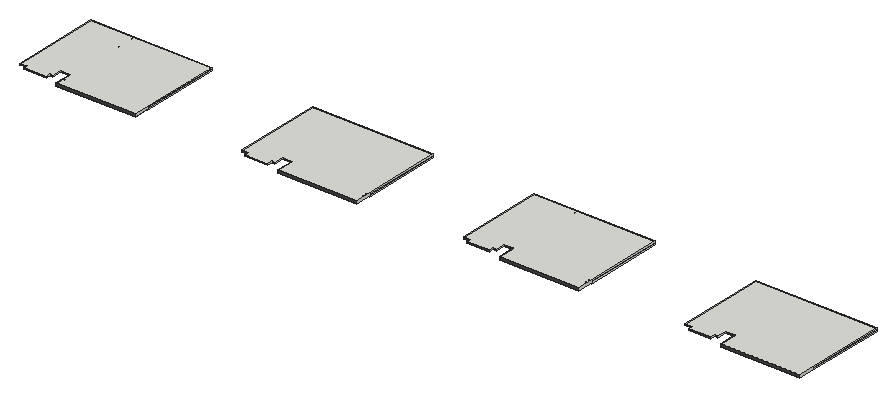
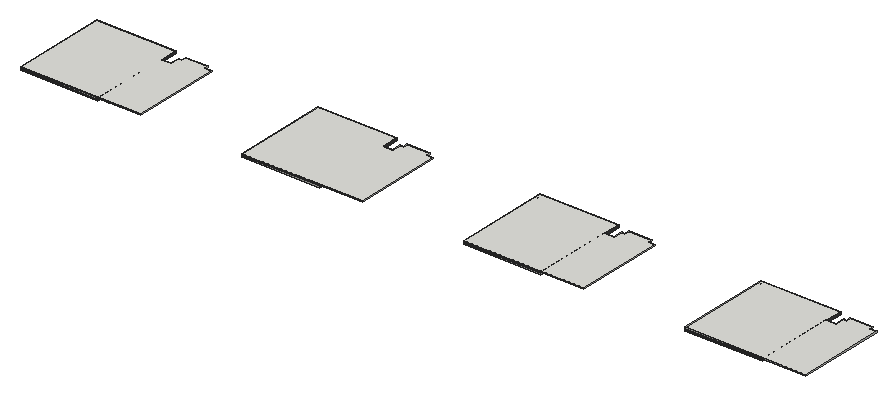
# SketchUp Ruby script. Lengths in inches.
U = 1.inch
M = Sketchup.active_model
def pt(a) = Geom::Point3d.new(a.map { |v| v * U })
def face(e, loops, mat)
  f = e.add_face(loops[0].map { |a| pt(a) })
  loops[1..].each { |l| e.add_face(l.map { |a| pt(a) }).erase! }
  f.material = f.back_material = mat if mat
  f
end
# faces: each face lists its corners as indices into pts; further lists are holes
def faces(e, pts, list, mat = nil) = list.each { |f| face(e, (f[0].is_a?(Array) ? f : [f]).map { |l| l.map { |i| pts[i] } }, mat) }
# xy, xz, yz: faces in a plane at the given z, y or x. An outline is a flat list of corners, or four numbers for a rectangle; further outlines are holes
def ring(l) = l.size == 4 ? [[l[0], l[1]], [l[2], l[1]], [l[2], l[3]], [l[0], l[3]]] : l.each_slice(2).to_a
def flat(e, list, mat, &to3) = list.each { |f| face(e, (f[0].is_a?(Array) ? f : [f]).map { |l| ring(l).map { |u, v| to3.(u, v) } }, mat) }
def xy(e, z, list, mat = nil) = flat(e, list, mat) { |x, y| [x, y, z] }
def xz(e, y, list, mat = nil) = flat(e, list, mat) { |x, z| [x, y, z] }
def yz(e, x, list, mat = nil) = flat(e, list, mat) { |y, z| [x, y, z] }
def lines(e, pts, list) = list.each { |a, b| e.add_line(pt(pts[a]), pt(pts[b])) }
# prism: a flat outline (further loops are holes) pulled along v
def prism(e, loops, v, mat = nil)
  f = face(e, loops, mat); d = Geom::Vector3d.new(v.map { |x| x * U })
  f.pushpull(f.normal.samedirection?(d) ? d.length : -d.length)
end
def box(e, o, s, mat = nil) = prism(e, [[o, [o[0] + s[0], o[1], o[2]], [o[0] + s[0], o[1] + s[1], o[2]], [o[0], o[1] + s[1], o[2]]]], [0, 0, s[2]], mat)
def at(x, y, z, deg = 0) = Geom::Transformation.translation(pt([x, y, z])) * Geom::Transformation.rotation(ORIGIN, Z_AXIS, deg.degrees)
def axes(o, x, y, z) = Geom::Transformation.new([*x, 0, *y, 0, *z, 0, *pt(o).to_a, 1])
def part(name) = M.definitions.add(name)
# library, detail: a bought-in or finely detailed component or shape, given as its bounding box
def library(name, o, s) = part(name).tap { |d| box(d.entities, o, s) }
def detail(e, o, s) = box(e.add_group.entities, o, s)
def put(e, d, t, mat = nil) = e.add_instance(d, t).tap { |i| i.material = mat if mat }
def group(e, t, mat = nil) = e.add_group.tap { |g| g.transformation = t; g.material = mat if mat }.entities
root = M.entities
M.materials.add("[Granite Dark Gray]").color = [69, 68, 68]
M.materials.add("[Mosaic Hexagonal Tile]").color = [48, 55, 63]
xy(root,776.0625,[[543.03,559.875,551.76,576.96],[551.76,559.875,990.19,576.96],[1793.65,559.875,1802.38,576.96],[1802.38,559.875,2240.81,576.96],[3044.28,559.875,3053.01,576.96],
  [3053.01,559.875,3491.44,576.96],[4294.9,559.875,4303.63,576.96],[4303.63,559.875,4742.06,576.96],[543.03,576.96,551.76,640.11],[977.59,576.96,990.19,651.03],
  [1793.65,576.96,1802.38,640.11],[2228.22,576.96,2240.81,651.03],[3044.28,576.96,3053.01,640.11],[3478.84,576.96,3491.44,651.03],[4294.9,576.96,4303.63,640.11],
  [4729.47,576.96,4742.06,651.03]],"[Granite Dark Gray]")
xy(root,784.4375,[[551.76,576.96,977.59,576.96,977.59,651.03,814.68,651.03,814.68,648.85,805.57,648.85,805.57,651.03,801.81,651.03,801.81,648.85,792.69,648.85,792.69,651.03,789.43,651.03,789.43,648.85,780.32,648.85,780.32,651.03,777.31,651.03,777.31,648.85,768.19,648.85,768.19,651.03,764.56,651.03,764.56,647.91,755.44,647.91,755.44,651.03,751.56,651.03,751.56,647.91,742.44,647.91,742.44,651.03,551.76,651.03],[1802.38,576.96,2228.22,576.96,2228.22,651.03,2065.31,651.03,2065.31,648.85,2056.19,648.85,2056.19,651.03,2052.43,651.03,2052.43,648.85,2043.32,648.85,2043.32,651.03,2040.06,651.03,2040.06,648.85,2030.94,648.85,2030.94,651.03,2027.93,651.03,2027.93,648.85,2018.82,648.85,2018.82,651.03,2015.18,651.03,2015.18,647.91,2006.07,647.91,2006.07,651.03,2002.18,651.03,2002.18,647.91,1993.07,647.91,1993.07,651.03,1802.38,651.03],[3053.01,576.96,3478.84,576.96,3478.84,651.03,3315.93,651.03,3315.93,648.85,3306.82,648.85,3306.82,651.03,3303.06,651.03,3303.06,648.85,3293.94,648.85,3293.94,651.03,3290.68,651.03,3290.68,648.85,3281.57,648.85,3281.57,651.03,3278.56,651.03,3278.56,648.85,3269.44,648.85,3269.44,651.03,3265.81,651.03,3265.81,647.91,3256.69,647.91,3256.69,651.03,3252.81,651.03,3252.81,647.91,3243.69,647.91,3243.69,651.03,3053.01,651.03],[4303.63,576.96,4729.47,576.96,4729.47,651.03,4566.56,651.03,4566.56,648.85,4557.44,648.85,4557.44,651.03,4553.68,651.03,4553.68,648.85,4544.57,648.85,4544.57,651.03,4541.31,651.03,4541.31,648.85,4532.19,648.85,4532.19,651.03,4529.18,651.03,4529.18,648.85,4520.07,648.85,4520.07,651.03,4516.43,651.03,4516.43,647.91,4507.32,647.91,4507.32,651.03,4503.43,651.03,4503.43,647.91,4494.32,647.91,4494.32,651.03,4303.63,651.03],[351.59,589.17,354.34,613.74],
  [354.34,589.17,464.1,613.74],[1602.22,589.17,1604.97,613.74],[1604.97,589.17,1714.72,613.74],[2852.84,589.17,2855.59,613.74],[2855.59,589.17,2965.35,613.74],
  [4103.47,589.17,4106.22,613.74],[4106.22,589.17,4215.97,613.74],[[310,613.74,482.97,1096.5],[341.26,653.8,475.14,1088.67]],[482.97,613.74,492.21,656.57],[[1560.62,613.74,1733.59,1096.5],[1591.89,653.8,1725.77,1088.67]],
  [1733.59,613.74,1742.84,656.57],[[2811.25,613.74,2984.22,1096.5],[2842.51,653.8,2976.39,1088.67]],[2984.22,613.74,2993.46,656.57],[[4061.87,613.74,4234.84,1096.5],[4093.14,653.8,4227.02,1088.67]],[4234.84,613.74,4244.09,656.57],
  [543.03,640.11,551.76,1096.5],[1793.65,640.11,1802.38,1096.5],[3044.28,640.11,3053.01,1096.5],[4294.9,640.11,4303.63,1096.5],[551.76,651.03,990.19,1096.5],
  [1802.38,651.03,2240.81,1096.5],[3053.01,651.03,3491.44,1096.5],[4303.63,651.03,4742.06,1096.5],[482.97,656.57,492.21,1096.5],[492.21,656.57,543.03,665.86],
  [1733.59,656.57,1742.84,1096.5],[1742.84,656.57,1793.65,665.86],[2984.22,656.57,2993.46,1096.5],[2993.46,656.57,3044.28,665.86],[4234.84,656.57,4244.09,1096.5],
  [4244.09,656.57,4294.9,665.86],[492.21,1079.1875,543.03,1096.5],[1742.84,1079.1875,1793.65,1096.5],[2993.46,1079.1875,3044.28,1096.5],[4244.09,1079.1875,4294.9,1096.5]])
xy(root,784.4375,[[345.68,577.92,345.68,598.8,310,598.8,310,613.74,351.59,613.74,351.59,589.17,464.1,589.17,464.1,577.92],[464.1,577.92,464.1,613.74,492.21,613.74,492.21,603.49,473.53,603.49,473.53,577.92],[1596.31,577.92,1596.31,598.8,1560.62,598.8,1560.62,613.74,1602.22,613.74,1602.22,589.17,1714.72,589.17,1714.72,577.92],[1714.72,577.92,1714.72,613.74,1742.84,613.74,1742.84,603.49,1724.16,603.49,1724.16,577.92],[2846.93,577.92,2846.93,598.8,2811.25,598.8,2811.25,613.74,2852.84,613.74,2852.84,589.17,2965.35,589.17,2965.35,577.92],
  [2965.35,577.92,2965.35,613.74,2993.46,613.74,2993.46,603.49,2974.78,603.49,2974.78,577.92],[4097.56,577.92,4097.56,598.8,4061.87,598.8,4061.87,613.74,4103.47,613.74,4103.47,589.17,4215.97,589.17,4215.97,577.92],[4215.97,577.92,4215.97,613.74,4244.09,613.74,4244.09,603.49,4225.41,603.49,4225.41,577.92]],"[Granite Dark Gray]")
xy(root,784.4375,[[492.21,665.86,543.03,1079.1875],[1742.84,665.86,1793.65,1079.1875],[2993.46,665.86,3044.28,1079.1875],[4244.09,665.86,4294.9,1079.1875]],"[Mosaic Hexagonal Tile]")
xy(root,785.86,[[351.59,585.86,354.34,589.17],[1602.22,585.86,1604.97,589.17],[2852.84,585.86,2855.59,589.17],[4103.47,585.86,4106.22,589.17]])
xy(root,790.4375,[[543.03,559.875,990.19,559.875,990.19,1096.5,310,1096.5,310,598.8,345.68,598.8,345.68,577.92,473.53,577.92,473.53,603.49,492.21,603.49,492.21,656.57,543.03,656.57],[1793.65,559.875,2240.81,559.875,2240.81,1096.5,1560.62,1096.5,1560.62,598.8,1596.31,598.8,1596.31,577.92,1724.16,577.92,1724.16,603.49,1742.84,603.49,1742.84,656.57,1793.65,656.57],[3044.28,559.875,3491.44,559.875,3491.44,1096.5,2811.25,1096.5,2811.25,598.8,2846.93,598.8,2846.93,577.92,2974.78,577.92,2974.78,603.49,2993.46,603.49,2993.46,656.57,3044.28,656.57],[4294.9,559.875,4742.06,559.875,4742.06,1096.5,4061.87,1096.5,4061.87,598.8,4097.56,598.8,4097.56,577.92,4225.41,577.92,4225.41,603.49,4244.09,603.49,4244.09,656.57,4294.9,656.57]])
xz(root,559.875,[[543.03,776.0625,990.19,790.4375],[1793.65,776.0625,2240.81,790.4375],[3044.28,776.0625,3491.44,790.4375],[4294.9,776.0625,4742.06,790.4375]],"[Granite Dark Gray]")
xz(root,576.96,[[551.76,776.0625,977.59,784.4375],[1802.38,776.0625,2228.22,784.4375],[3053.01,776.0625,3478.84,784.4375],[4303.63,776.0625,4729.47,784.4375]])
xz(root,577.92,[[345.68,784.4375,473.53,790.4375],[1596.31,784.4375,1724.16,790.4375],[2846.93,784.4375,2974.78,790.4375],[4097.56,784.4375,4225.41,790.4375]],"[Granite Dark Gray]")
xz(root,589.17,[[351.59,784.4375,354.34,785.86],[1602.22,784.4375,1604.97,785.86],[2852.84,784.4375,2855.59,785.86],[4103.47,784.4375,4106.22,785.86]])
xz(root,598.8,[[310,784.4375,345.68,790.4375],[1560.62,784.4375,1596.31,790.4375],[2811.25,784.4375,2846.93,790.4375],[4061.87,784.4375,4097.56,790.4375]],"[Granite Dark Gray]")
xz(root,603.49,[[473.53,784.4375,492.21,790.4375],[1724.16,784.4375,1742.84,790.4375],[2974.78,784.4375,2993.46,790.4375],[4225.41,784.4375,4244.09,790.4375]],"[Granite Dark Gray]")
xz(root,640.11,[[543.03,776.0625,551.76,784.4375],[1793.65,776.0625,1802.38,784.4375],[3044.28,776.0625,3053.01,784.4375],[4294.9,776.0625,4303.63,784.4375]])
xz(root,651.03,[[551.76,772.4375,563.08,778.4375],[978.86,772.4375,990.19,776.0625],[1802.38,772.4375,1813.71,778.4375],[2229.49,772.4375,2240.81,776.0625],[3053.01,772.4375,3064.33,778.4375],
  [3480.11,772.4375,3491.44,776.0625],[4303.63,772.4375,4314.96,778.4375],[4730.74,772.4375,4742.06,776.0625],[977.59,776.0625,978.86,778.4375],[978.86,776.0625,990.19,778.4375],
  [2228.22,776.0625,2229.49,778.4375],[2229.49,776.0625,2240.81,778.4375],[3478.84,776.0625,3480.11,778.4375],[3480.11,776.0625,3491.44,778.4375],[4729.47,776.0625,4730.74,778.4375],
  [4730.74,776.0625,4742.06,778.4375],[977.59,778.4375,990.19,784.4375],[2228.22,778.4375,2240.81,784.4375],[3478.84,778.4375,3491.44,784.4375],[4729.47,778.4375,4742.06,784.4375]])
xz(root,656.57,[[492.21,784.4375,543.03,790.4375],[1742.84,784.4375,1793.65,790.4375],[2993.46,784.4375,3044.28,790.4375],[4244.09,784.4375,4294.9,790.4375]],"[Granite Dark Gray]")
xz(root,657.03,[[563.08,772.4375,978.86,778.4375],[1813.71,772.4375,2229.49,778.4375],[3064.33,772.4375,3480.11,778.4375],[4314.96,772.4375,4730.74,778.4375]])
xz(root,1085.17,[[563.08,772.4375,978.86,778.4375],[1813.71,772.4375,2229.49,778.4375],[3064.33,772.4375,3480.11,778.4375],[4314.96,772.4375,4730.74,778.4375]])
xz(root,1096.5,[[551.76,772.4375,990.19,778.4375],[1802.38,772.4375,2240.81,778.4375],[3053.01,772.4375,3491.44,778.4375],[4303.63,772.4375,4742.06,778.4375],[551.76,778.4375,990.19,784.4375],
  [1802.38,778.4375,2240.81,784.4375],[3053.01,778.4375,3491.44,784.4375],[4303.63,778.4375,4742.06,784.4375],[310,784.4375,990.19,790.4375],[1560.62,784.4375,2240.81,790.4375],
  [2811.25,784.4375,3491.44,790.4375],[4061.87,784.4375,4742.06,790.4375]])
yz(root,310,[[598.8,784.4375,1096.5,790.4375]])
yz(root,345.68,[[577.92,784.4375,598.8,790.4375]])
yz(root,473.53,[[577.92,784.4375,603.49,790.4375]])
yz(root,492.21,[[603.49,784.4375,656.57,790.4375]])
yz(root,543.03,[[559.875,776.0625,559.875,790.4375,656.57,790.4375,656.57,784.4375,640.11,784.4375,640.11,776.0625]],"[Granite Dark Gray]")
yz(root,551.76,[[651.03,772.4375,1096.5,778.4375],[576.96,776.0625,640.11,784.4375],[651.03,778.4375,1096.5,784.4375]])
yz(root,563.08,[[657.03,772.4375,1085.17,778.4375]])
yz(root,977.59,[[576.96,776.0625,651.03,784.4375]])
yz(root,978.86,[[657.03,772.4375,1085.17,778.4375]])
yz(root,990.19,[[651.03,772.4375,1096.5,778.4375],[559.875,776.0625,651.03,776.0625,651.03,784.4375,1096.5,784.4375,1096.5,790.4375,559.875,790.4375],[651.03,778.4375,1096.5,784.4375]])
yz(root,1560.62,[[598.8,784.4375,1096.5,790.4375]])
yz(root,1596.31,[[577.92,784.4375,598.8,790.4375]])
yz(root,1724.16,[[577.92,784.4375,603.49,790.4375]])
yz(root,1742.84,[[603.49,784.4375,656.57,790.4375]])
yz(root,1793.65,[[559.875,776.0625,559.875,790.4375,656.57,790.4375,656.57,784.4375,640.11,784.4375,640.11,776.0625]],"[Granite Dark Gray]")
yz(root,1802.38,[[651.03,772.4375,1096.5,778.4375],[576.96,776.0625,640.11,784.4375],[651.03,778.4375,1096.5,784.4375]])
yz(root,1813.71,[[657.03,772.4375,1085.17,778.4375]])
yz(root,2228.22,[[576.96,776.0625,651.03,784.4375]])
yz(root,2229.49,[[657.03,772.4375,1085.17,778.4375]])
yz(root,2240.81,[[651.03,772.4375,1096.5,778.4375],[559.875,776.0625,651.03,776.0625,651.03,784.4375,1096.5,784.4375,1096.5,790.4375,559.875,790.4375],[651.03,778.4375,1096.5,784.4375]])
yz(root,2811.25,[[598.8,784.4375,1096.5,790.4375]])
yz(root,2846.93,[[577.92,784.4375,598.8,790.4375]])
yz(root,2974.78,[[577.92,784.4375,603.49,790.4375]])
yz(root,2993.46,[[603.49,784.4375,656.57,790.4375]])
yz(root,3044.28,[[559.875,776.0625,559.875,790.4375,656.57,790.4375,656.57,784.4375,640.11,784.4375,640.11,776.0625]],"[Granite Dark Gray]")
yz(root,3053.01,[[651.03,772.4375,1096.5,778.4375],[576.96,776.0625,640.11,784.4375],[651.03,778.4375,1096.5,784.4375]])
yz(root,3064.33,[[657.03,772.4375,1085.17,778.4375]])
yz(root,3478.84,[[576.96,776.0625,651.03,784.4375]])
yz(root,3480.11,[[657.03,772.4375,1085.17,778.4375]])
yz(root,3491.44,[[651.03,772.4375,1096.5,778.4375],[559.875,776.0625,651.03,776.0625,651.03,784.4375,1096.5,784.4375,1096.5,790.4375,559.875,790.4375],[651.03,778.4375,1096.5,784.4375]])
yz(root,4061.87,[[598.8,784.4375,1096.5,790.4375]])
yz(root,4097.56,[[577.92,784.4375,598.8,790.4375]])
yz(root,4225.41,[[577.92,784.4375,603.49,790.4375]])
yz(root,4244.09,[[603.49,784.4375,656.57,790.4375]])
yz(root,4294.9,[[559.875,776.0625,559.875,790.4375,656.57,790.4375,656.57,784.4375,640.11,784.4375,640.11,776.0625]],"[Granite Dark Gray]")
yz(root,4303.63,[[651.03,772.4375,1096.5,778.4375],[576.96,776.0625,640.11,784.4375],[651.03,778.4375,1096.5,784.4375]])
yz(root,4314.96,[[657.03,772.4375,1085.17,778.4375]])
yz(root,4729.47,[[576.96,776.0625,651.03,784.4375]])
yz(root,4730.74,[[657.03,772.4375,1085.17,778.4375]])
yz(root,4742.06,[[651.03,772.4375,1096.5,778.4375],[559.875,776.0625,651.03,776.0625,651.03,784.4375,1096.5,784.4375,1096.5,790.4375,559.875,790.4375],[651.03,778.4375,1096.5,784.4375]])
p = [[2846.93,598.8,784.4375],[2846.93,603.49,784.4375],[4097.56,598.8,784.4375],[4097.56,603.49,784.4375],[345.68,598.8,784.4375],[345.68,603.49,784.4375],
  [1596.31,598.8,784.4375],[1596.31,603.49,784.4375]]
lines(root,p,[[0,1],[2,3],[4,5],[6,7]])
